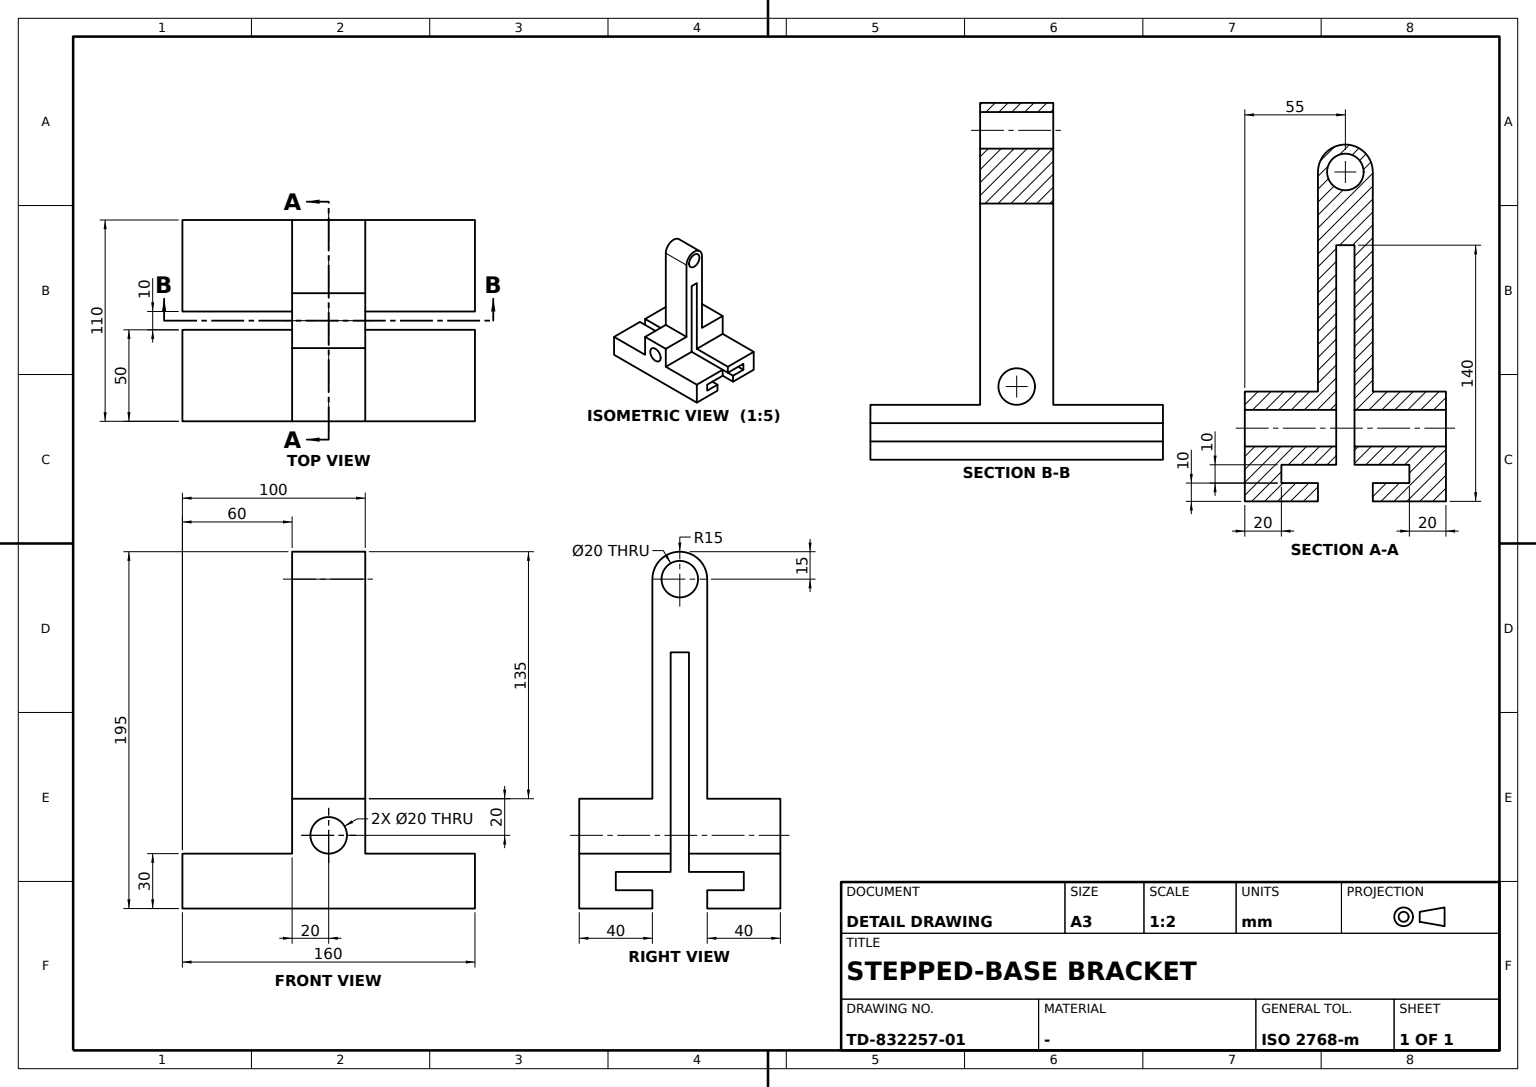
ISO-10303-21;
HEADER;
FILE_DESCRIPTION((''),'2;1');
FILE_NAME('','',(''),(''),'','','');
FILE_SCHEMA(('AUTOMOTIVE_DESIGN'));
ENDSEC;
DATA;
#1=APPLICATION_CONTEXT('');
#2=PRODUCT_CONTEXT('',#1,'mechanical');
#3=PRODUCT('','','',(#2));
#4=PRODUCT_DEFINITION_FORMATION('','',#3);
#5=PRODUCT_DEFINITION_CONTEXT('',#1,'design');
#6=PRODUCT_DEFINITION('','',#4,#5);
#7=PRODUCT_DEFINITION_SHAPE('','',#6);
#8=(LENGTH_UNIT()NAMED_UNIT(*)SI_UNIT(.MILLI.,.METRE.));
#9=(NAMED_UNIT(*)PLANE_ANGLE_UNIT()SI_UNIT($,.RADIAN.));
#10=(NAMED_UNIT(*)SI_UNIT($,.STERADIAN.)SOLID_ANGLE_UNIT());
#11=UNCERTAINTY_MEASURE_WITH_UNIT(LENGTH_MEASURE(1.E-05),#8,'distance_accuracy_value','');
#12=(GEOMETRIC_REPRESENTATION_CONTEXT(3)GLOBAL_UNCERTAINTY_ASSIGNED_CONTEXT((#11))GLOBAL_UNIT_ASSIGNED_CONTEXT((#8,#9,#10))REPRESENTATION_CONTEXT('',''));
#13=CARTESIAN_POINT('',(-80.,35.,-20.));
#14=VERTEX_POINT('',#13);
#15=CARTESIAN_POINT('',(-80.,15.,-20.));
#16=VERTEX_POINT('',#15);
#17=CARTESIAN_POINT('',(-80.,25.,-20.));
#18=DIRECTION('',(0.,-1.,0.));
#19=VECTOR('',#18,1000.);
#20=LINE('',#17,#19);
#21=EDGE_CURVE('',#14,#16,#20,.T.);
#22=ORIENTED_EDGE('',*,*,#21,.T.);
#23=CARTESIAN_POINT('',(80.,15.,-20.));
#24=VERTEX_POINT('',#23);
#25=CARTESIAN_POINT('',(0.,15.,-20.));
#26=DIRECTION('',(1.,0.,0.));
#27=VECTOR('',#26,1000.);
#28=LINE('',#25,#27);
#29=EDGE_CURVE('',#16,#24,#28,.T.);
#30=ORIENTED_EDGE('',*,*,#29,.T.);
#31=CARTESIAN_POINT('',(80.,35.,-20.));
#32=VERTEX_POINT('',#31);
#33=CARTESIAN_POINT('',(80.,25.,-20.));
#34=LINE('',#33,#19);
#35=EDGE_CURVE('',#32,#24,#34,.T.);
#36=ORIENTED_EDGE('',*,*,#35,.F.);
#37=CARTESIAN_POINT('',(0.,35.,-20.));
#38=LINE('',#37,#27);
#39=EDGE_CURVE('',#14,#32,#38,.T.);
#40=ORIENTED_EDGE('',*,*,#39,.F.);
#41=EDGE_LOOP('',(#22,#30,#36,#40));
#42=FACE_OUTER_BOUND('',#41,.T.);
#43=CARTESIAN_POINT('',(0.,-15.,-20.));
#44=DIRECTION('',(0.,0.,1.));
#45=AXIS2_PLACEMENT_3D('',#43,#44,#18);
#46=PLANE('',#45);
#47=ADVANCED_FACE('',(#42),#46,.T.);
#48=CARTESIAN_POINT('',(-20.,-10.,150.));
#49=VERTEX_POINT('',#48);
#50=CARTESIAN_POINT('',(20.,-10.,150.));
#51=VERTEX_POINT('',#50);
#52=CARTESIAN_POINT('',(0.,-10.,150.));
#53=LINE('',#52,#27);
#54=EDGE_CURVE('',#49,#51,#53,.T.);
#55=ORIENTED_EDGE('',*,*,#54,.F.);
#56=CARTESIAN_POINT('',(-20.,10.,150.));
#57=VERTEX_POINT('',#56);
#58=CARTESIAN_POINT('',(-20.,0.,150.));
#59=DIRECTION('',(0.,1.,0.));
#60=AXIS2_PLACEMENT_3D('',#58,#26,#59);
#61=CIRCLE('',#60,10.);
#62=EDGE_CURVE('',#57,#49,#61,.T.);
#63=ORIENTED_EDGE('',*,*,#62,.F.);
#64=CARTESIAN_POINT('',(20.,10.,150.));
#65=VERTEX_POINT('',#64);
#66=CARTESIAN_POINT('',(0.,10.,150.));
#67=LINE('',#66,#27);
#68=EDGE_CURVE('',#57,#65,#67,.T.);
#69=ORIENTED_EDGE('',*,*,#68,.T.);
#70=CARTESIAN_POINT('',(20.,0.,150.));
#71=AXIS2_PLACEMENT_3D('',#70,#26,#59);
#72=CIRCLE('',#71,10.);
#73=EDGE_CURVE('',#65,#51,#72,.T.);
#74=ORIENTED_EDGE('',*,*,#73,.T.);
#75=EDGE_LOOP('',(#55,#63,#69,#74));
#76=FACE_OUTER_BOUND('',#75,.T.);
#77=CARTESIAN_POINT('',(0.,0.,150.));
#78=DIRECTION('',(-1.,0.,0.));
#79=AXIS2_PLACEMENT_3D('',#77,#78,#59);
#80=CYLINDRICAL_SURFACE('',#79,10.);
#81=ADVANCED_FACE('',(#76),#80,.F.);
#82=CARTESIAN_POINT('',(10.,55.,10.));
#83=VERTEX_POINT('',#82);
#84=CARTESIAN_POINT('',(-10.,55.,10.));
#85=VERTEX_POINT('',#84);
#86=CARTESIAN_POINT('',(0.,55.,10.));
#87=AXIS2_PLACEMENT_3D('',#86,#59,#78);
#88=CIRCLE('',#87,10.);
#89=EDGE_CURVE('',#83,#85,#88,.T.);
#90=ORIENTED_EDGE('',*,*,#89,.F.);
#91=EDGE_CURVE('',#85,#83,#88,.T.);
#92=ORIENTED_EDGE('',*,*,#91,.F.);
#93=EDGE_LOOP('',(#90,#92));
#94=FACE_BOUND('',#93,.T.);
#95=CARTESIAN_POINT('',(-80.,55.,-30.));
#96=VERTEX_POINT('',#95);
#97=CARTESIAN_POINT('',(-80.,55.,0.));
#98=VERTEX_POINT('',#97);
#99=CARTESIAN_POINT('',(-80.,55.,-15.));
#100=VECTOR('',#44,1000.);
#101=LINE('',#99,#100);
#102=EDGE_CURVE('',#96,#98,#101,.T.);
#103=ORIENTED_EDGE('',*,*,#102,.T.);
#104=CARTESIAN_POINT('',(-20.,55.,0.));
#105=VERTEX_POINT('',#104);
#106=CARTESIAN_POINT('',(-50.,55.,0.));
#107=LINE('',#106,#27);
#108=EDGE_CURVE('',#98,#105,#107,.T.);
#109=ORIENTED_EDGE('',*,*,#108,.T.);
#110=CARTESIAN_POINT('',(-20.,55.,30.));
#111=VERTEX_POINT('',#110);
#112=CARTESIAN_POINT('',(-20.,55.,15.));
#113=LINE('',#112,#100);
#114=EDGE_CURVE('',#105,#111,#113,.T.);
#115=ORIENTED_EDGE('',*,*,#114,.T.);
#116=CARTESIAN_POINT('',(20.,55.,30.));
#117=VERTEX_POINT('',#116);
#118=CARTESIAN_POINT('',(0.,55.,30.));
#119=LINE('',#118,#27);
#120=EDGE_CURVE('',#111,#117,#119,.T.);
#121=ORIENTED_EDGE('',*,*,#120,.T.);
#122=CARTESIAN_POINT('',(20.,55.,0.));
#123=VERTEX_POINT('',#122);
#124=CARTESIAN_POINT('',(20.,55.,15.));
#125=LINE('',#124,#100);
#126=EDGE_CURVE('',#123,#117,#125,.T.);
#127=ORIENTED_EDGE('',*,*,#126,.F.);
#128=CARTESIAN_POINT('',(80.,55.,0.));
#129=VERTEX_POINT('',#128);
#130=CARTESIAN_POINT('',(50.,55.,0.));
#131=LINE('',#130,#27);
#132=EDGE_CURVE('',#123,#129,#131,.T.);
#133=ORIENTED_EDGE('',*,*,#132,.T.);
#134=CARTESIAN_POINT('',(80.,55.,-30.));
#135=VERTEX_POINT('',#134);
#136=CARTESIAN_POINT('',(80.,55.,-15.));
#137=LINE('',#136,#100);
#138=EDGE_CURVE('',#135,#129,#137,.T.);
#139=ORIENTED_EDGE('',*,*,#138,.F.);
#140=CARTESIAN_POINT('',(0.,55.,-30.));
#141=LINE('',#140,#27);
#142=EDGE_CURVE('',#96,#135,#141,.T.);
#143=ORIENTED_EDGE('',*,*,#142,.F.);
#144=EDGE_LOOP('',(#103,#109,#115,#121,#127,#133,#139,#143));
#145=FACE_OUTER_BOUND('',#144,.T.);
#146=CARTESIAN_POINT('',(0.,55.,0.));
#147=DIRECTION('',(0.,0.,-1.));
#148=AXIS2_PLACEMENT_3D('',#146,#18,#147);
#149=PLANE('',#148);
#150=ADVANCED_FACE('',(#94,#145),#149,.F.);
#151=CARTESIAN_POINT('',(10.,-5.,10.));
#152=VERTEX_POINT('',#151);
#153=CARTESIAN_POINT('',(10.,-55.,10.));
#154=VERTEX_POINT('',#153);
#155=CARTESIAN_POINT('',(10.,-0.66,10.));
#156=LINE('',#155,#19);
#157=EDGE_CURVE('',#152,#154,#156,.T.);
#158=ORIENTED_EDGE('',*,*,#157,.F.);
#159=CARTESIAN_POINT('',(-10.,-5.,10.));
#160=VERTEX_POINT('',#159);
#161=CARTESIAN_POINT('',(0.,-5.,10.));
#162=AXIS2_PLACEMENT_3D('',#161,#59,#44);
#163=CIRCLE('',#162,10.);
#164=EDGE_CURVE('',#152,#160,#163,.T.);
#165=ORIENTED_EDGE('',*,*,#164,.T.);
#166=CARTESIAN_POINT('',(-10.,-55.,10.));
#167=VERTEX_POINT('',#166);
#168=CARTESIAN_POINT('',(-10.,-0.66,10.));
#169=LINE('',#168,#19);
#170=EDGE_CURVE('',#160,#167,#169,.T.);
#171=ORIENTED_EDGE('',*,*,#170,.T.);
#172=CARTESIAN_POINT('',(0.,-55.,10.));
#173=AXIS2_PLACEMENT_3D('',#172,#18,#147);
#174=CIRCLE('',#173,10.);
#175=EDGE_CURVE('',#167,#154,#174,.T.);
#176=ORIENTED_EDGE('',*,*,#175,.T.);
#177=EDGE_LOOP('',(#158,#165,#171,#176));
#178=FACE_OUTER_BOUND('',#177,.T.);
#179=CARTESIAN_POINT('',(0.,-0.66,10.));
#180=AXIS2_PLACEMENT_3D('',#179,#18,#78);
#181=CYLINDRICAL_SURFACE('',#180,10.);
#182=ADVANCED_FACE('',(#178),#181,.F.);
#183=CARTESIAN_POINT('',(-80.,-55.,0.));
#184=VERTEX_POINT('',#183);
#185=CARTESIAN_POINT('',(-80.,-55.,-30.));
#186=VERTEX_POINT('',#185);
#187=CARTESIAN_POINT('',(-80.,-55.,-15.));
#188=VECTOR('',#147,1000.);
#189=LINE('',#187,#188);
#190=EDGE_CURVE('',#184,#186,#189,.T.);
#191=ORIENTED_EDGE('',*,*,#190,.T.);
#192=CARTESIAN_POINT('',(80.,-55.,-30.));
#193=VERTEX_POINT('',#192);
#194=CARTESIAN_POINT('',(0.,-55.,-30.));
#195=LINE('',#194,#27);
#196=EDGE_CURVE('',#186,#193,#195,.T.);
#197=ORIENTED_EDGE('',*,*,#196,.T.);
#198=CARTESIAN_POINT('',(80.,-55.,0.));
#199=VERTEX_POINT('',#198);
#200=CARTESIAN_POINT('',(80.,-55.,-15.));
#201=LINE('',#200,#188);
#202=EDGE_CURVE('',#199,#193,#201,.T.);
#203=ORIENTED_EDGE('',*,*,#202,.F.);
#204=CARTESIAN_POINT('',(20.,-55.,0.));
#205=VERTEX_POINT('',#204);
#206=CARTESIAN_POINT('',(50.,-55.,0.));
#207=LINE('',#206,#27);
#208=EDGE_CURVE('',#205,#199,#207,.T.);
#209=ORIENTED_EDGE('',*,*,#208,.F.);
#210=CARTESIAN_POINT('',(20.,-55.,30.));
#211=VERTEX_POINT('',#210);
#212=CARTESIAN_POINT('',(20.,-55.,15.));
#213=LINE('',#212,#188);
#214=EDGE_CURVE('',#211,#205,#213,.T.);
#215=ORIENTED_EDGE('',*,*,#214,.F.);
#216=CARTESIAN_POINT('',(-20.,-55.,30.));
#217=VERTEX_POINT('',#216);
#218=CARTESIAN_POINT('',(0.,-55.,30.));
#219=LINE('',#218,#27);
#220=EDGE_CURVE('',#217,#211,#219,.T.);
#221=ORIENTED_EDGE('',*,*,#220,.F.);
#222=CARTESIAN_POINT('',(-20.,-55.,0.));
#223=VERTEX_POINT('',#222);
#224=CARTESIAN_POINT('',(-20.,-55.,15.));
#225=LINE('',#224,#188);
#226=EDGE_CURVE('',#217,#223,#225,.T.);
#227=ORIENTED_EDGE('',*,*,#226,.T.);
#228=CARTESIAN_POINT('',(-50.,-55.,0.));
#229=LINE('',#228,#27);
#230=EDGE_CURVE('',#184,#223,#229,.T.);
#231=ORIENTED_EDGE('',*,*,#230,.F.);
#232=EDGE_LOOP('',(#191,#197,#203,#209,#215,#221,#227,#231));
#233=FACE_OUTER_BOUND('',#232,.T.);
#234=EDGE_CURVE('',#154,#167,#174,.T.);
#235=ORIENTED_EDGE('',*,*,#234,.F.);
#236=ORIENTED_EDGE('',*,*,#175,.F.);
#237=EDGE_LOOP('',(#235,#236));
#238=FACE_BOUND('',#237,.T.);
#239=CARTESIAN_POINT('',(0.,-55.,0.));
#240=AXIS2_PLACEMENT_3D('',#239,#18,#147);
#241=PLANE('',#240);
#242=ADVANCED_FACE('',(#233,#238),#241,.T.);
#243=ORIENTED_EDGE('',*,*,#62,.T.);
#244=EDGE_CURVE('',#49,#57,#61,.T.);
#245=ORIENTED_EDGE('',*,*,#244,.T.);
#246=EDGE_LOOP('',(#243,#245));
#247=FACE_BOUND('',#246,.T.);
#248=ORIENTED_EDGE('',*,*,#114,.F.);
#249=CARTESIAN_POINT('',(-20.,5.,0.));
#250=VERTEX_POINT('',#249);
#251=CARTESIAN_POINT('',(-20.,30.,0.));
#252=VECTOR('',#59,1000.);
#253=LINE('',#251,#252);
#254=EDGE_CURVE('',#250,#105,#253,.T.);
#255=ORIENTED_EDGE('',*,*,#254,.F.);
#256=CARTESIAN_POINT('',(-20.,5.,110.));
#257=VERTEX_POINT('',#256);
#258=CARTESIAN_POINT('',(-20.,5.,55.));
#259=LINE('',#258,#188);
#260=EDGE_CURVE('',#257,#250,#259,.T.);
#261=ORIENTED_EDGE('',*,*,#260,.F.);
#262=CARTESIAN_POINT('',(-20.,-5.,110.));
#263=VERTEX_POINT('',#262);
#264=CARTESIAN_POINT('',(-20.,0.,110.));
#265=LINE('',#264,#252);
#266=EDGE_CURVE('',#263,#257,#265,.T.);
#267=ORIENTED_EDGE('',*,*,#266,.F.);
#268=CARTESIAN_POINT('',(-20.,-5.,0.));
#269=VERTEX_POINT('',#268);
#270=CARTESIAN_POINT('',(-20.,-5.,55.));
#271=LINE('',#270,#100);
#272=EDGE_CURVE('',#269,#263,#271,.T.);
#273=ORIENTED_EDGE('',*,*,#272,.F.);
#274=CARTESIAN_POINT('',(-20.,-30.,0.));
#275=LINE('',#274,#252);
#276=EDGE_CURVE('',#223,#269,#275,.T.);
#277=ORIENTED_EDGE('',*,*,#276,.F.);
#278=ORIENTED_EDGE('',*,*,#226,.F.);
#279=CARTESIAN_POINT('',(-20.,-15.,30.));
#280=VERTEX_POINT('',#279);
#281=CARTESIAN_POINT('',(-20.,-35.,30.));
#282=LINE('',#281,#19);
#283=EDGE_CURVE('',#280,#217,#282,.T.);
#284=ORIENTED_EDGE('',*,*,#283,.F.);
#285=CARTESIAN_POINT('',(-20.,-15.,150.));
#286=VERTEX_POINT('',#285);
#287=CARTESIAN_POINT('',(-20.,-15.,90.));
#288=LINE('',#287,#188);
#289=EDGE_CURVE('',#286,#280,#288,.T.);
#290=ORIENTED_EDGE('',*,*,#289,.F.);
#291=CARTESIAN_POINT('',(-20.,15.,150.));
#292=VERTEX_POINT('',#291);
#293=CIRCLE('',#60,15.);
#294=EDGE_CURVE('',#292,#286,#293,.T.);
#295=ORIENTED_EDGE('',*,*,#294,.F.);
#296=CARTESIAN_POINT('',(-20.,15.,30.));
#297=VERTEX_POINT('',#296);
#298=CARTESIAN_POINT('',(-20.,15.,90.));
#299=LINE('',#298,#100);
#300=EDGE_CURVE('',#297,#292,#299,.T.);
#301=ORIENTED_EDGE('',*,*,#300,.F.);
#302=CARTESIAN_POINT('',(-20.,35.,30.));
#303=LINE('',#302,#19);
#304=EDGE_CURVE('',#111,#297,#303,.T.);
#305=ORIENTED_EDGE('',*,*,#304,.F.);
#306=EDGE_LOOP('',(#248,#255,#261,#267,#273,#277,#278,#284,#290,#295,#301,#305));
#307=FACE_OUTER_BOUND('',#306,.T.);
#308=CARTESIAN_POINT('',(-20.,0.,0.));
#309=AXIS2_PLACEMENT_3D('',#308,#26,#59);
#310=PLANE('',#309);
#311=ADVANCED_FACE('',(#247,#307),#310,.F.);
#312=CARTESIAN_POINT('',(20.,5.,0.));
#313=VERTEX_POINT('',#312);
#314=CARTESIAN_POINT('',(80.,5.,0.));
#315=VERTEX_POINT('',#314);
#316=CARTESIAN_POINT('',(50.,5.,0.));
#317=LINE('',#316,#27);
#318=EDGE_CURVE('',#313,#315,#317,.T.);
#319=ORIENTED_EDGE('',*,*,#318,.T.);
#320=CARTESIAN_POINT('',(80.,30.,0.));
#321=LINE('',#320,#19);
#322=EDGE_CURVE('',#129,#315,#321,.T.);
#323=ORIENTED_EDGE('',*,*,#322,.F.);
#324=ORIENTED_EDGE('',*,*,#132,.F.);
#325=CARTESIAN_POINT('',(20.,30.,0.));
#326=LINE('',#325,#252);
#327=EDGE_CURVE('',#313,#123,#326,.T.);
#328=ORIENTED_EDGE('',*,*,#327,.F.);
#329=EDGE_LOOP('',(#319,#323,#324,#328));
#330=FACE_OUTER_BOUND('',#329,.T.);
#331=CARTESIAN_POINT('',(0.,-5.,0.));
#332=AXIS2_PLACEMENT_3D('',#331,#44,#18);
#333=PLANE('',#332);
#334=ADVANCED_FACE('',(#330),#333,.T.);
#335=CARTESIAN_POINT('',(-80.,-15.,-30.));
#336=VERTEX_POINT('',#335);
#337=CARTESIAN_POINT('',(80.,-15.,-30.));
#338=VERTEX_POINT('',#337);
#339=CARTESIAN_POINT('',(0.,-15.,-30.));
#340=LINE('',#339,#27);
#341=EDGE_CURVE('',#336,#338,#340,.T.);
#342=ORIENTED_EDGE('',*,*,#341,.F.);
#343=CARTESIAN_POINT('',(-80.,-15.,-20.));
#344=VERTEX_POINT('',#343);
#345=CARTESIAN_POINT('',(-80.,-15.,-25.));
#346=LINE('',#345,#100);
#347=EDGE_CURVE('',#336,#344,#346,.T.);
#348=ORIENTED_EDGE('',*,*,#347,.T.);
#349=CARTESIAN_POINT('',(80.,-15.,-20.));
#350=VERTEX_POINT('',#349);
#351=LINE('',#43,#27);
#352=EDGE_CURVE('',#344,#350,#351,.T.);
#353=ORIENTED_EDGE('',*,*,#352,.T.);
#354=CARTESIAN_POINT('',(80.,-15.,-25.));
#355=LINE('',#354,#100);
#356=EDGE_CURVE('',#338,#350,#355,.T.);
#357=ORIENTED_EDGE('',*,*,#356,.F.);
#358=EDGE_LOOP('',(#342,#348,#353,#357));
#359=FACE_OUTER_BOUND('',#358,.T.);
#360=AXIS2_PLACEMENT_3D('',#339,#59,#44);
#361=PLANE('',#360);
#362=ADVANCED_FACE('',(#359),#361,.T.);
#363=ORIENTED_EDGE('',*,*,#347,.F.);
#364=CARTESIAN_POINT('',(-80.,-35.,-30.));
#365=LINE('',#364,#252);
#366=EDGE_CURVE('',#186,#336,#365,.T.);
#367=ORIENTED_EDGE('',*,*,#366,.F.);
#368=ORIENTED_EDGE('',*,*,#190,.F.);
#369=CARTESIAN_POINT('',(-80.,-5.,0.));
#370=VERTEX_POINT('',#369);
#371=CARTESIAN_POINT('',(-80.,-30.,0.));
#372=LINE('',#371,#19);
#373=EDGE_CURVE('',#370,#184,#372,.T.);
#374=ORIENTED_EDGE('',*,*,#373,.F.);
#375=CARTESIAN_POINT('',(-80.,-5.,-10.));
#376=VERTEX_POINT('',#375);
#377=CARTESIAN_POINT('',(-80.,-5.,-5.));
#378=LINE('',#377,#100);
#379=EDGE_CURVE('',#376,#370,#378,.T.);
#380=ORIENTED_EDGE('',*,*,#379,.F.);
#381=CARTESIAN_POINT('',(-80.,-35.,-10.));
#382=VERTEX_POINT('',#381);
#383=CARTESIAN_POINT('',(-80.,-20.,-10.));
#384=LINE('',#383,#252);
#385=EDGE_CURVE('',#382,#376,#384,.T.);
#386=ORIENTED_EDGE('',*,*,#385,.F.);
#387=CARTESIAN_POINT('',(-80.,-35.,-20.));
#388=VERTEX_POINT('',#387);
#389=CARTESIAN_POINT('',(-80.,-35.,-15.));
#390=LINE('',#389,#100);
#391=EDGE_CURVE('',#388,#382,#390,.T.);
#392=ORIENTED_EDGE('',*,*,#391,.F.);
#393=CARTESIAN_POINT('',(-80.,-25.,-20.));
#394=LINE('',#393,#19);
#395=EDGE_CURVE('',#344,#388,#394,.T.);
#396=ORIENTED_EDGE('',*,*,#395,.F.);
#397=EDGE_LOOP('',(#363,#367,#368,#374,#380,#386,#392,#396));
#398=FACE_OUTER_BOUND('',#397,.T.);
#399=CARTESIAN_POINT('',(-80.,0.,0.));
#400=AXIS2_PLACEMENT_3D('',#399,#26,#59);
#401=PLANE('',#400);
#402=ADVANCED_FACE('',(#398),#401,.F.);
#403=CARTESIAN_POINT('',(-80.,5.,-10.));
#404=VERTEX_POINT('',#403);
#405=CARTESIAN_POINT('',(-80.,35.,-10.));
#406=VERTEX_POINT('',#405);
#407=CARTESIAN_POINT('',(-80.,20.,-10.));
#408=LINE('',#407,#252);
#409=EDGE_CURVE('',#404,#406,#408,.T.);
#410=ORIENTED_EDGE('',*,*,#409,.F.);
#411=CARTESIAN_POINT('',(-80.,5.,0.));
#412=VERTEX_POINT('',#411);
#413=CARTESIAN_POINT('',(-80.,5.,-5.));
#414=LINE('',#413,#188);
#415=EDGE_CURVE('',#412,#404,#414,.T.);
#416=ORIENTED_EDGE('',*,*,#415,.F.);
#417=CARTESIAN_POINT('',(-80.,30.,0.));
#418=LINE('',#417,#19);
#419=EDGE_CURVE('',#98,#412,#418,.T.);
#420=ORIENTED_EDGE('',*,*,#419,.F.);
#421=ORIENTED_EDGE('',*,*,#102,.F.);
#422=CARTESIAN_POINT('',(-80.,15.,-30.));
#423=VERTEX_POINT('',#422);
#424=CARTESIAN_POINT('',(-80.,35.,-30.));
#425=LINE('',#424,#252);
#426=EDGE_CURVE('',#423,#96,#425,.T.);
#427=ORIENTED_EDGE('',*,*,#426,.F.);
#428=CARTESIAN_POINT('',(-80.,15.,-25.));
#429=LINE('',#428,#188);
#430=EDGE_CURVE('',#16,#423,#429,.T.);
#431=ORIENTED_EDGE('',*,*,#430,.F.);
#432=ORIENTED_EDGE('',*,*,#21,.F.);
#433=CARTESIAN_POINT('',(-80.,35.,-15.));
#434=LINE('',#433,#188);
#435=EDGE_CURVE('',#406,#14,#434,.T.);
#436=ORIENTED_EDGE('',*,*,#435,.F.);
#437=EDGE_LOOP('',(#410,#416,#420,#421,#427,#431,#432,#436));
#438=FACE_OUTER_BOUND('',#437,.T.);
#439=ADVANCED_FACE('',(#438),#401,.F.);
#440=ORIENTED_EDGE('',*,*,#352,.F.);
#441=ORIENTED_EDGE('',*,*,#395,.T.);
#442=CARTESIAN_POINT('',(80.,-35.,-20.));
#443=VERTEX_POINT('',#442);
#444=CARTESIAN_POINT('',(0.,-35.,-20.));
#445=LINE('',#444,#27);
#446=EDGE_CURVE('',#388,#443,#445,.T.);
#447=ORIENTED_EDGE('',*,*,#446,.T.);
#448=CARTESIAN_POINT('',(80.,-25.,-20.));
#449=LINE('',#448,#19);
#450=EDGE_CURVE('',#350,#443,#449,.T.);
#451=ORIENTED_EDGE('',*,*,#450,.F.);
#452=EDGE_LOOP('',(#440,#441,#447,#451));
#453=FACE_OUTER_BOUND('',#452,.T.);
#454=ADVANCED_FACE('',(#453),#46,.T.);
#455=CARTESIAN_POINT('',(-50.,5.,0.));
#456=LINE('',#455,#27);
#457=EDGE_CURVE('',#412,#250,#456,.T.);
#458=ORIENTED_EDGE('',*,*,#457,.T.);
#459=ORIENTED_EDGE('',*,*,#254,.T.);
#460=ORIENTED_EDGE('',*,*,#108,.F.);
#461=ORIENTED_EDGE('',*,*,#419,.T.);
#462=EDGE_LOOP('',(#458,#459,#460,#461));
#463=FACE_OUTER_BOUND('',#462,.T.);
#464=ADVANCED_FACE('',(#463),#333,.T.);
#465=CARTESIAN_POINT('',(80.,-35.,-10.));
#466=VERTEX_POINT('',#465);
#467=CARTESIAN_POINT('',(80.,-5.,-10.));
#468=VERTEX_POINT('',#467);
#469=CARTESIAN_POINT('',(80.,-20.,-10.));
#470=LINE('',#469,#252);
#471=EDGE_CURVE('',#466,#468,#470,.T.);
#472=ORIENTED_EDGE('',*,*,#471,.F.);
#473=CARTESIAN_POINT('',(0.,-35.,-10.));
#474=LINE('',#473,#27);
#475=EDGE_CURVE('',#382,#466,#474,.T.);
#476=ORIENTED_EDGE('',*,*,#475,.F.);
#477=ORIENTED_EDGE('',*,*,#385,.T.);
#478=CARTESIAN_POINT('',(0.,-5.,-10.));
#479=LINE('',#478,#27);
#480=EDGE_CURVE('',#376,#468,#479,.T.);
#481=ORIENTED_EDGE('',*,*,#480,.T.);
#482=EDGE_LOOP('',(#472,#476,#477,#481));
#483=FACE_OUTER_BOUND('',#482,.T.);
#484=AXIS2_PLACEMENT_3D('',#473,#147,#59);
#485=PLANE('',#484);
#486=ADVANCED_FACE('',(#483),#485,.T.);
#487=ORIENTED_EDGE('',*,*,#170,.F.);
#488=EDGE_CURVE('',#160,#152,#163,.T.);
#489=ORIENTED_EDGE('',*,*,#488,.T.);
#490=ORIENTED_EDGE('',*,*,#157,.T.);
#491=ORIENTED_EDGE('',*,*,#234,.T.);
#492=EDGE_LOOP('',(#487,#489,#490,#491));
#493=FACE_OUTER_BOUND('',#492,.T.);
#494=ADVANCED_FACE('',(#493),#181,.F.);
#495=CARTESIAN_POINT('',(80.,15.,-30.));
#496=VERTEX_POINT('',#495);
#497=CARTESIAN_POINT('',(80.,35.,-30.));
#498=LINE('',#497,#252);
#499=EDGE_CURVE('',#496,#135,#498,.T.);
#500=ORIENTED_EDGE('',*,*,#499,.F.);
#501=CARTESIAN_POINT('',(0.,15.,-30.));
#502=LINE('',#501,#27);
#503=EDGE_CURVE('',#423,#496,#502,.T.);
#504=ORIENTED_EDGE('',*,*,#503,.F.);
#505=ORIENTED_EDGE('',*,*,#426,.T.);
#506=ORIENTED_EDGE('',*,*,#142,.T.);
#507=EDGE_LOOP('',(#500,#504,#505,#506));
#508=FACE_OUTER_BOUND('',#507,.T.);
#509=AXIS2_PLACEMENT_3D('',#194,#147,#59);
#510=PLANE('',#509);
#511=ADVANCED_FACE('',(#508),#510,.T.);
#512=ORIENTED_EDGE('',*,*,#68,.F.);
#513=ORIENTED_EDGE('',*,*,#244,.F.);
#514=ORIENTED_EDGE('',*,*,#54,.T.);
#515=EDGE_CURVE('',#51,#65,#72,.T.);
#516=ORIENTED_EDGE('',*,*,#515,.T.);
#517=EDGE_LOOP('',(#512,#513,#514,#516));
#518=FACE_OUTER_BOUND('',#517,.T.);
#519=ADVANCED_FACE('',(#518),#80,.F.);
#520=CARTESIAN_POINT('',(20.,15.,150.));
#521=VERTEX_POINT('',#520);
#522=CARTESIAN_POINT('',(0.,15.,150.));
#523=LINE('',#522,#27);
#524=EDGE_CURVE('',#292,#521,#523,.T.);
#525=ORIENTED_EDGE('',*,*,#524,.T.);
#526=CARTESIAN_POINT('',(20.,15.,30.));
#527=VERTEX_POINT('',#526);
#528=CARTESIAN_POINT('',(20.,15.,90.));
#529=LINE('',#528,#100);
#530=EDGE_CURVE('',#527,#521,#529,.T.);
#531=ORIENTED_EDGE('',*,*,#530,.F.);
#532=CARTESIAN_POINT('',(0.,15.,30.));
#533=LINE('',#532,#27);
#534=EDGE_CURVE('',#297,#527,#533,.T.);
#535=ORIENTED_EDGE('',*,*,#534,.F.);
#536=ORIENTED_EDGE('',*,*,#300,.T.);
#537=EDGE_LOOP('',(#525,#531,#535,#536));
#538=FACE_OUTER_BOUND('',#537,.T.);
#539=AXIS2_PLACEMENT_3D('',#501,#59,#44);
#540=PLANE('',#539);
#541=ADVANCED_FACE('',(#538),#540,.T.);
#542=CARTESIAN_POINT('',(-10.,5.,10.));
#543=VERTEX_POINT('',#542);
#544=CARTESIAN_POINT('',(10.,5.,10.));
#545=VERTEX_POINT('',#544);
#546=CARTESIAN_POINT('',(0.,5.,10.));
#547=AXIS2_PLACEMENT_3D('',#546,#59,#44);
#548=CIRCLE('',#547,10.);
#549=EDGE_CURVE('',#543,#545,#548,.T.);
#550=ORIENTED_EDGE('',*,*,#549,.T.);
#551=EDGE_CURVE('',#545,#543,#548,.T.);
#552=ORIENTED_EDGE('',*,*,#551,.T.);
#553=EDGE_LOOP('',(#550,#552));
#554=FACE_BOUND('',#553,.T.);
#555=ORIENTED_EDGE('',*,*,#260,.T.);
#556=ORIENTED_EDGE('',*,*,#457,.F.);
#557=ORIENTED_EDGE('',*,*,#415,.T.);
#558=CARTESIAN_POINT('',(80.,5.,-10.));
#559=VERTEX_POINT('',#558);
#560=CARTESIAN_POINT('',(0.,5.,-10.));
#561=LINE('',#560,#27);
#562=EDGE_CURVE('',#404,#559,#561,.T.);
#563=ORIENTED_EDGE('',*,*,#562,.T.);
#564=CARTESIAN_POINT('',(80.,5.,-5.));
#565=LINE('',#564,#188);
#566=EDGE_CURVE('',#315,#559,#565,.T.);
#567=ORIENTED_EDGE('',*,*,#566,.F.);
#568=ORIENTED_EDGE('',*,*,#318,.F.);
#569=CARTESIAN_POINT('',(20.,5.,110.));
#570=VERTEX_POINT('',#569);
#571=CARTESIAN_POINT('',(20.,5.,55.));
#572=LINE('',#571,#188);
#573=EDGE_CURVE('',#570,#313,#572,.T.);
#574=ORIENTED_EDGE('',*,*,#573,.F.);
#575=CARTESIAN_POINT('',(0.,5.,110.));
#576=LINE('',#575,#27);
#577=EDGE_CURVE('',#257,#570,#576,.T.);
#578=ORIENTED_EDGE('',*,*,#577,.F.);
#579=EDGE_LOOP('',(#555,#556,#557,#563,#567,#568,#574,#578));
#580=FACE_OUTER_BOUND('',#579,.T.);
#581=AXIS2_PLACEMENT_3D('',#560,#59,#44);
#582=PLANE('',#581);
#583=ADVANCED_FACE('',(#554,#580),#582,.F.);
#584=CARTESIAN_POINT('',(80.,35.,-10.));
#585=VERTEX_POINT('',#584);
#586=CARTESIAN_POINT('',(80.,35.,-15.));
#587=LINE('',#586,#188);
#588=EDGE_CURVE('',#585,#32,#587,.T.);
#589=ORIENTED_EDGE('',*,*,#588,.F.);
#590=CARTESIAN_POINT('',(0.,35.,-10.));
#591=LINE('',#590,#27);
#592=EDGE_CURVE('',#406,#585,#591,.T.);
#593=ORIENTED_EDGE('',*,*,#592,.F.);
#594=ORIENTED_EDGE('',*,*,#435,.T.);
#595=ORIENTED_EDGE('',*,*,#39,.T.);
#596=EDGE_LOOP('',(#589,#593,#594,#595));
#597=FACE_OUTER_BOUND('',#596,.T.);
#598=AXIS2_PLACEMENT_3D('',#37,#59,#44);
#599=PLANE('',#598);
#600=ADVANCED_FACE('',(#597),#599,.F.);
#601=CARTESIAN_POINT('',(20.,-5.,0.));
#602=VERTEX_POINT('',#601);
#603=CARTESIAN_POINT('',(20.,-5.,110.));
#604=VERTEX_POINT('',#603);
#605=CARTESIAN_POINT('',(20.,-5.,55.));
#606=LINE('',#605,#100);
#607=EDGE_CURVE('',#602,#604,#606,.T.);
#608=ORIENTED_EDGE('',*,*,#607,.F.);
#609=CARTESIAN_POINT('',(80.,-5.,0.));
#610=VERTEX_POINT('',#609);
#611=CARTESIAN_POINT('',(50.,-5.,0.));
#612=LINE('',#611,#27);
#613=EDGE_CURVE('',#602,#610,#612,.T.);
#614=ORIENTED_EDGE('',*,*,#613,.T.);
#615=CARTESIAN_POINT('',(80.,-5.,-5.));
#616=LINE('',#615,#100);
#617=EDGE_CURVE('',#468,#610,#616,.T.);
#618=ORIENTED_EDGE('',*,*,#617,.F.);
#619=ORIENTED_EDGE('',*,*,#480,.F.);
#620=ORIENTED_EDGE('',*,*,#379,.T.);
#621=CARTESIAN_POINT('',(-50.,-5.,0.));
#622=LINE('',#621,#27);
#623=EDGE_CURVE('',#370,#269,#622,.T.);
#624=ORIENTED_EDGE('',*,*,#623,.T.);
#625=ORIENTED_EDGE('',*,*,#272,.T.);
#626=CARTESIAN_POINT('',(0.,-5.,110.));
#627=LINE('',#626,#27);
#628=EDGE_CURVE('',#263,#604,#627,.T.);
#629=ORIENTED_EDGE('',*,*,#628,.T.);
#630=EDGE_LOOP('',(#608,#614,#618,#619,#620,#624,#625,#629));
#631=FACE_OUTER_BOUND('',#630,.T.);
#632=ORIENTED_EDGE('',*,*,#488,.F.);
#633=ORIENTED_EDGE('',*,*,#164,.F.);
#634=EDGE_LOOP('',(#632,#633));
#635=FACE_BOUND('',#634,.T.);
#636=AXIS2_PLACEMENT_3D('',#478,#59,#44);
#637=PLANE('',#636);
#638=ADVANCED_FACE('',(#631,#635),#637,.T.);
#639=ORIENTED_EDGE('',*,*,#577,.T.);
#640=CARTESIAN_POINT('',(20.,0.,110.));
#641=LINE('',#640,#252);
#642=EDGE_CURVE('',#604,#570,#641,.T.);
#643=ORIENTED_EDGE('',*,*,#642,.F.);
#644=ORIENTED_EDGE('',*,*,#628,.F.);
#645=ORIENTED_EDGE('',*,*,#266,.T.);
#646=EDGE_LOOP('',(#639,#643,#644,#645));
#647=FACE_OUTER_BOUND('',#646,.T.);
#648=AXIS2_PLACEMENT_3D('',#626,#147,#59);
#649=PLANE('',#648);
#650=ADVANCED_FACE('',(#647),#649,.T.);
#651=CARTESIAN_POINT('',(80.,20.,-10.));
#652=LINE('',#651,#252);
#653=EDGE_CURVE('',#559,#585,#652,.T.);
#654=ORIENTED_EDGE('',*,*,#653,.T.);
#655=ORIENTED_EDGE('',*,*,#588,.T.);
#656=ORIENTED_EDGE('',*,*,#35,.T.);
#657=CARTESIAN_POINT('',(80.,15.,-25.));
#658=LINE('',#657,#188);
#659=EDGE_CURVE('',#24,#496,#658,.T.);
#660=ORIENTED_EDGE('',*,*,#659,.T.);
#661=ORIENTED_EDGE('',*,*,#499,.T.);
#662=ORIENTED_EDGE('',*,*,#138,.T.);
#663=ORIENTED_EDGE('',*,*,#322,.T.);
#664=ORIENTED_EDGE('',*,*,#566,.T.);
#665=EDGE_LOOP('',(#654,#655,#656,#660,#661,#662,#663,#664));
#666=FACE_OUTER_BOUND('',#665,.T.);
#667=CARTESIAN_POINT('',(80.,0.,0.));
#668=AXIS2_PLACEMENT_3D('',#667,#26,#59);
#669=PLANE('',#668);
#670=ADVANCED_FACE('',(#666),#669,.T.);
#671=ORIENTED_EDGE('',*,*,#659,.F.);
#672=ORIENTED_EDGE('',*,*,#29,.F.);
#673=ORIENTED_EDGE('',*,*,#430,.T.);
#674=ORIENTED_EDGE('',*,*,#503,.T.);
#675=EDGE_LOOP('',(#671,#672,#673,#674));
#676=FACE_OUTER_BOUND('',#675,.T.);
#677=ADVANCED_FACE('',(#676),#540,.F.);
#678=ORIENTED_EDGE('',*,*,#446,.F.);
#679=ORIENTED_EDGE('',*,*,#391,.T.);
#680=ORIENTED_EDGE('',*,*,#475,.T.);
#681=CARTESIAN_POINT('',(80.,-35.,-15.));
#682=LINE('',#681,#100);
#683=EDGE_CURVE('',#443,#466,#682,.T.);
#684=ORIENTED_EDGE('',*,*,#683,.F.);
#685=EDGE_LOOP('',(#678,#679,#680,#684));
#686=FACE_OUTER_BOUND('',#685,.T.);
#687=AXIS2_PLACEMENT_3D('',#444,#59,#44);
#688=PLANE('',#687);
#689=ADVANCED_FACE('',(#686),#688,.T.);
#690=ORIENTED_EDGE('',*,*,#208,.T.);
#691=CARTESIAN_POINT('',(80.,-30.,0.));
#692=LINE('',#691,#19);
#693=EDGE_CURVE('',#610,#199,#692,.T.);
#694=ORIENTED_EDGE('',*,*,#693,.F.);
#695=ORIENTED_EDGE('',*,*,#613,.F.);
#696=CARTESIAN_POINT('',(20.,-30.,0.));
#697=LINE('',#696,#252);
#698=EDGE_CURVE('',#205,#602,#697,.T.);
#699=ORIENTED_EDGE('',*,*,#698,.F.);
#700=EDGE_LOOP('',(#690,#694,#695,#699));
#701=FACE_OUTER_BOUND('',#700,.T.);
#702=ADVANCED_FACE('',(#701),#333,.T.);
#703=ORIENTED_EDGE('',*,*,#693,.T.);
#704=ORIENTED_EDGE('',*,*,#202,.T.);
#705=CARTESIAN_POINT('',(80.,-35.,-30.));
#706=LINE('',#705,#252);
#707=EDGE_CURVE('',#193,#338,#706,.T.);
#708=ORIENTED_EDGE('',*,*,#707,.T.);
#709=ORIENTED_EDGE('',*,*,#356,.T.);
#710=ORIENTED_EDGE('',*,*,#450,.T.);
#711=ORIENTED_EDGE('',*,*,#683,.T.);
#712=ORIENTED_EDGE('',*,*,#471,.T.);
#713=ORIENTED_EDGE('',*,*,#617,.T.);
#714=EDGE_LOOP('',(#703,#704,#708,#709,#710,#711,#712,#713));
#715=FACE_OUTER_BOUND('',#714,.T.);
#716=ADVANCED_FACE('',(#715),#669,.T.);
#717=CARTESIAN_POINT('',(20.,-15.,30.));
#718=VERTEX_POINT('',#717);
#719=CARTESIAN_POINT('',(0.,-15.,30.));
#720=LINE('',#719,#27);
#721=EDGE_CURVE('',#280,#718,#720,.T.);
#722=ORIENTED_EDGE('',*,*,#721,.F.);
#723=ORIENTED_EDGE('',*,*,#283,.T.);
#724=ORIENTED_EDGE('',*,*,#220,.T.);
#725=CARTESIAN_POINT('',(20.,-35.,30.));
#726=LINE('',#725,#19);
#727=EDGE_CURVE('',#718,#211,#726,.T.);
#728=ORIENTED_EDGE('',*,*,#727,.F.);
#729=EDGE_LOOP('',(#722,#723,#724,#728));
#730=FACE_OUTER_BOUND('',#729,.T.);
#731=AXIS2_PLACEMENT_3D('',#118,#44,#18);
#732=PLANE('',#731);
#733=ADVANCED_FACE('',(#730),#732,.T.);
#734=ORIENTED_EDGE('',*,*,#230,.T.);
#735=ORIENTED_EDGE('',*,*,#276,.T.);
#736=ORIENTED_EDGE('',*,*,#623,.F.);
#737=ORIENTED_EDGE('',*,*,#373,.T.);
#738=EDGE_LOOP('',(#734,#735,#736,#737));
#739=FACE_OUTER_BOUND('',#738,.T.);
#740=ADVANCED_FACE('',(#739),#333,.T.);
#741=EDGE_CURVE('',#83,#545,#156,.T.);
#742=ORIENTED_EDGE('',*,*,#741,.F.);
#743=ORIENTED_EDGE('',*,*,#89,.T.);
#744=EDGE_CURVE('',#85,#543,#169,.T.);
#745=ORIENTED_EDGE('',*,*,#744,.T.);
#746=ORIENTED_EDGE('',*,*,#551,.F.);
#747=EDGE_LOOP('',(#742,#743,#745,#746));
#748=FACE_OUTER_BOUND('',#747,.T.);
#749=ADVANCED_FACE('',(#748),#181,.F.);
#750=CARTESIAN_POINT('',(20.,35.,30.));
#751=LINE('',#750,#19);
#752=EDGE_CURVE('',#117,#527,#751,.T.);
#753=ORIENTED_EDGE('',*,*,#752,.F.);
#754=ORIENTED_EDGE('',*,*,#120,.F.);
#755=ORIENTED_EDGE('',*,*,#304,.T.);
#756=ORIENTED_EDGE('',*,*,#534,.T.);
#757=EDGE_LOOP('',(#753,#754,#755,#756));
#758=FACE_OUTER_BOUND('',#757,.T.);
#759=ADVANCED_FACE('',(#758),#732,.T.);
#760=ORIENTED_EDGE('',*,*,#294,.T.);
#761=CARTESIAN_POINT('',(20.,-15.,150.));
#762=VERTEX_POINT('',#761);
#763=CARTESIAN_POINT('',(0.,-15.,150.));
#764=LINE('',#763,#27);
#765=EDGE_CURVE('',#286,#762,#764,.T.);
#766=ORIENTED_EDGE('',*,*,#765,.T.);
#767=CIRCLE('',#71,15.);
#768=EDGE_CURVE('',#521,#762,#767,.T.);
#769=ORIENTED_EDGE('',*,*,#768,.F.);
#770=ORIENTED_EDGE('',*,*,#524,.F.);
#771=EDGE_LOOP('',(#760,#766,#769,#770));
#772=FACE_OUTER_BOUND('',#771,.T.);
#773=CYLINDRICAL_SURFACE('',#79,15.);
#774=ADVANCED_FACE('',(#772),#773,.T.);
#775=ORIENTED_EDGE('',*,*,#707,.F.);
#776=ORIENTED_EDGE('',*,*,#196,.F.);
#777=ORIENTED_EDGE('',*,*,#366,.T.);
#778=ORIENTED_EDGE('',*,*,#341,.T.);
#779=EDGE_LOOP('',(#775,#776,#777,#778));
#780=FACE_OUTER_BOUND('',#779,.T.);
#781=ADVANCED_FACE('',(#780),#510,.T.);
#782=ORIENTED_EDGE('',*,*,#562,.F.);
#783=ORIENTED_EDGE('',*,*,#409,.T.);
#784=ORIENTED_EDGE('',*,*,#592,.T.);
#785=ORIENTED_EDGE('',*,*,#653,.F.);
#786=EDGE_LOOP('',(#782,#783,#784,#785));
#787=FACE_OUTER_BOUND('',#786,.T.);
#788=ADVANCED_FACE('',(#787),#485,.T.);
#789=ORIENTED_EDGE('',*,*,#289,.T.);
#790=ORIENTED_EDGE('',*,*,#721,.T.);
#791=CARTESIAN_POINT('',(20.,-15.,90.));
#792=LINE('',#791,#188);
#793=EDGE_CURVE('',#762,#718,#792,.T.);
#794=ORIENTED_EDGE('',*,*,#793,.F.);
#795=ORIENTED_EDGE('',*,*,#765,.F.);
#796=EDGE_LOOP('',(#789,#790,#794,#795));
#797=FACE_OUTER_BOUND('',#796,.T.);
#798=ADVANCED_FACE('',(#797),#361,.F.);
#799=ORIENTED_EDGE('',*,*,#515,.F.);
#800=ORIENTED_EDGE('',*,*,#73,.F.);
#801=EDGE_LOOP('',(#799,#800));
#802=FACE_BOUND('',#801,.T.);
#803=ORIENTED_EDGE('',*,*,#698,.T.);
#804=ORIENTED_EDGE('',*,*,#607,.T.);
#805=ORIENTED_EDGE('',*,*,#642,.T.);
#806=ORIENTED_EDGE('',*,*,#573,.T.);
#807=ORIENTED_EDGE('',*,*,#327,.T.);
#808=ORIENTED_EDGE('',*,*,#126,.T.);
#809=ORIENTED_EDGE('',*,*,#752,.T.);
#810=ORIENTED_EDGE('',*,*,#530,.T.);
#811=ORIENTED_EDGE('',*,*,#768,.T.);
#812=ORIENTED_EDGE('',*,*,#793,.T.);
#813=ORIENTED_EDGE('',*,*,#727,.T.);
#814=ORIENTED_EDGE('',*,*,#214,.T.);
#815=EDGE_LOOP('',(#803,#804,#805,#806,#807,#808,#809,#810,#811,#812,#813,#814));
#816=FACE_OUTER_BOUND('',#815,.T.);
#817=CARTESIAN_POINT('',(20.,0.,0.));
#818=AXIS2_PLACEMENT_3D('',#817,#26,#59);
#819=PLANE('',#818);
#820=ADVANCED_FACE('',(#802,#816),#819,.T.);
#821=ORIENTED_EDGE('',*,*,#549,.F.);
#822=ORIENTED_EDGE('',*,*,#744,.F.);
#823=ORIENTED_EDGE('',*,*,#91,.T.);
#824=ORIENTED_EDGE('',*,*,#741,.T.);
#825=EDGE_LOOP('',(#821,#822,#823,#824));
#826=FACE_OUTER_BOUND('',#825,.T.);
#827=ADVANCED_FACE('',(#826),#181,.F.);
#828=CLOSED_SHELL('',(#47,#81,#150,#182,#242,#311,#334,#362,#402,#439,#454,#464,#486,#494,#511,#519,#541,#583,#600,#638,#650,#670,#677,#689,#702,#716,#733,#740,#749,#759,#774,#781,#788,#798,#820,#827));
#829=MANIFOLD_SOLID_BREP('',#828);
#830=ADVANCED_BREP_SHAPE_REPRESENTATION('',(#829),#12);
#831=SHAPE_DEFINITION_REPRESENTATION(#7,#830);
ENDSEC;
END-ISO-10303-21;
